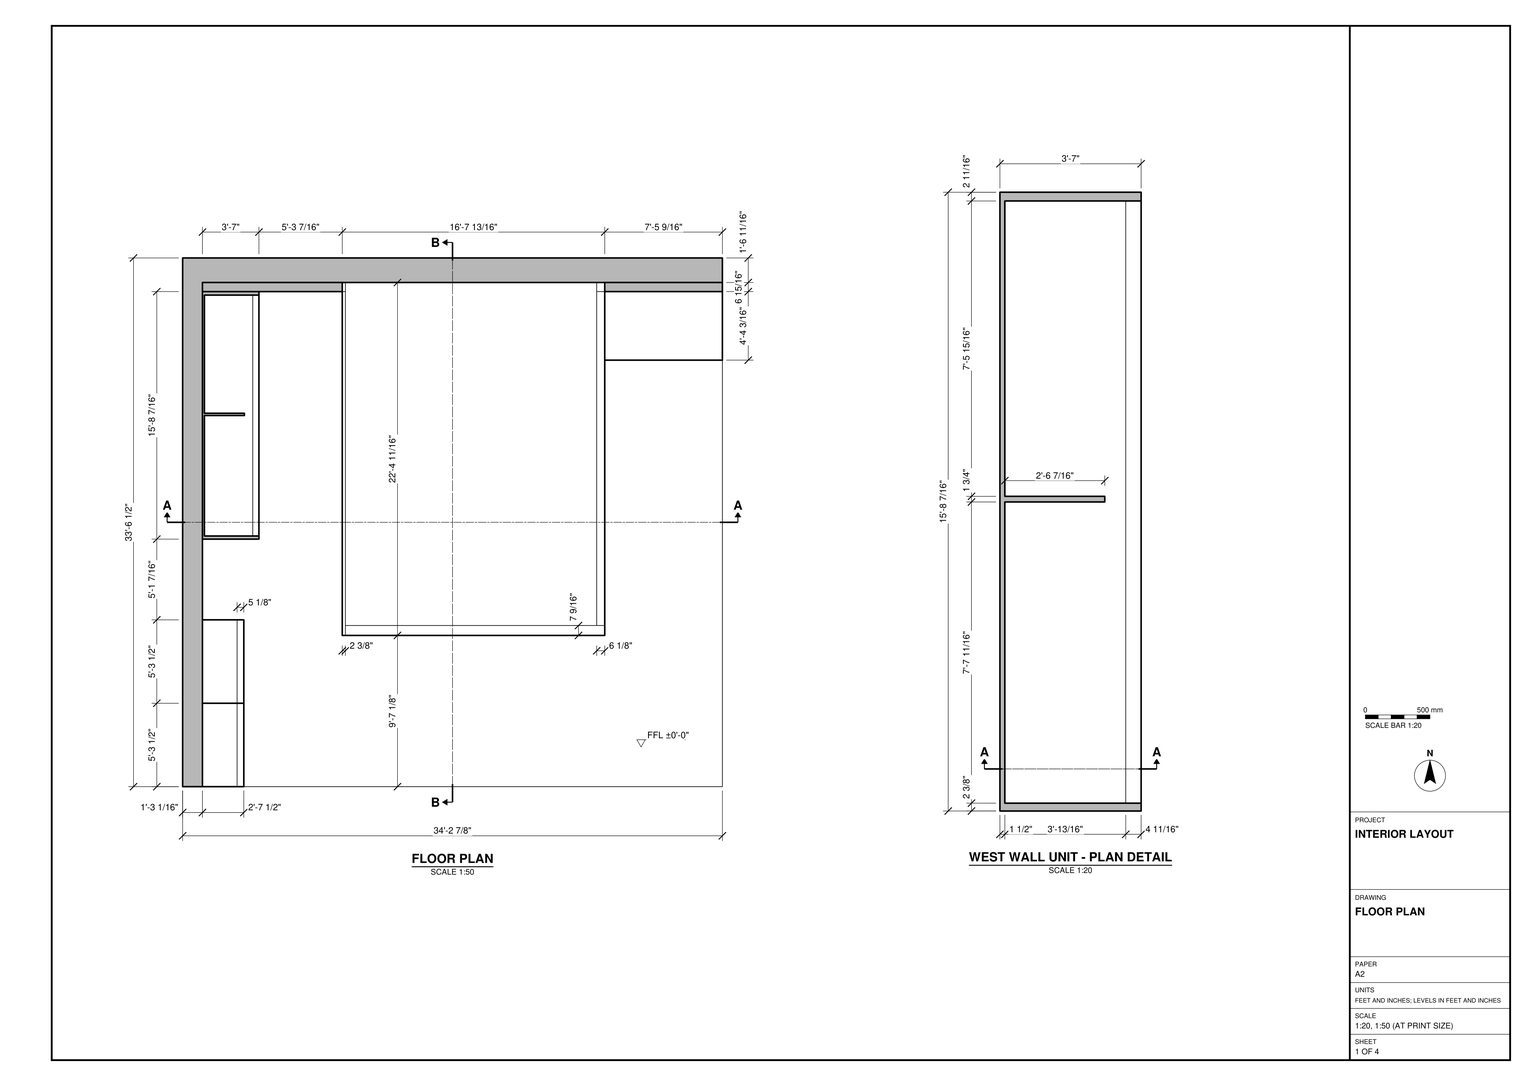
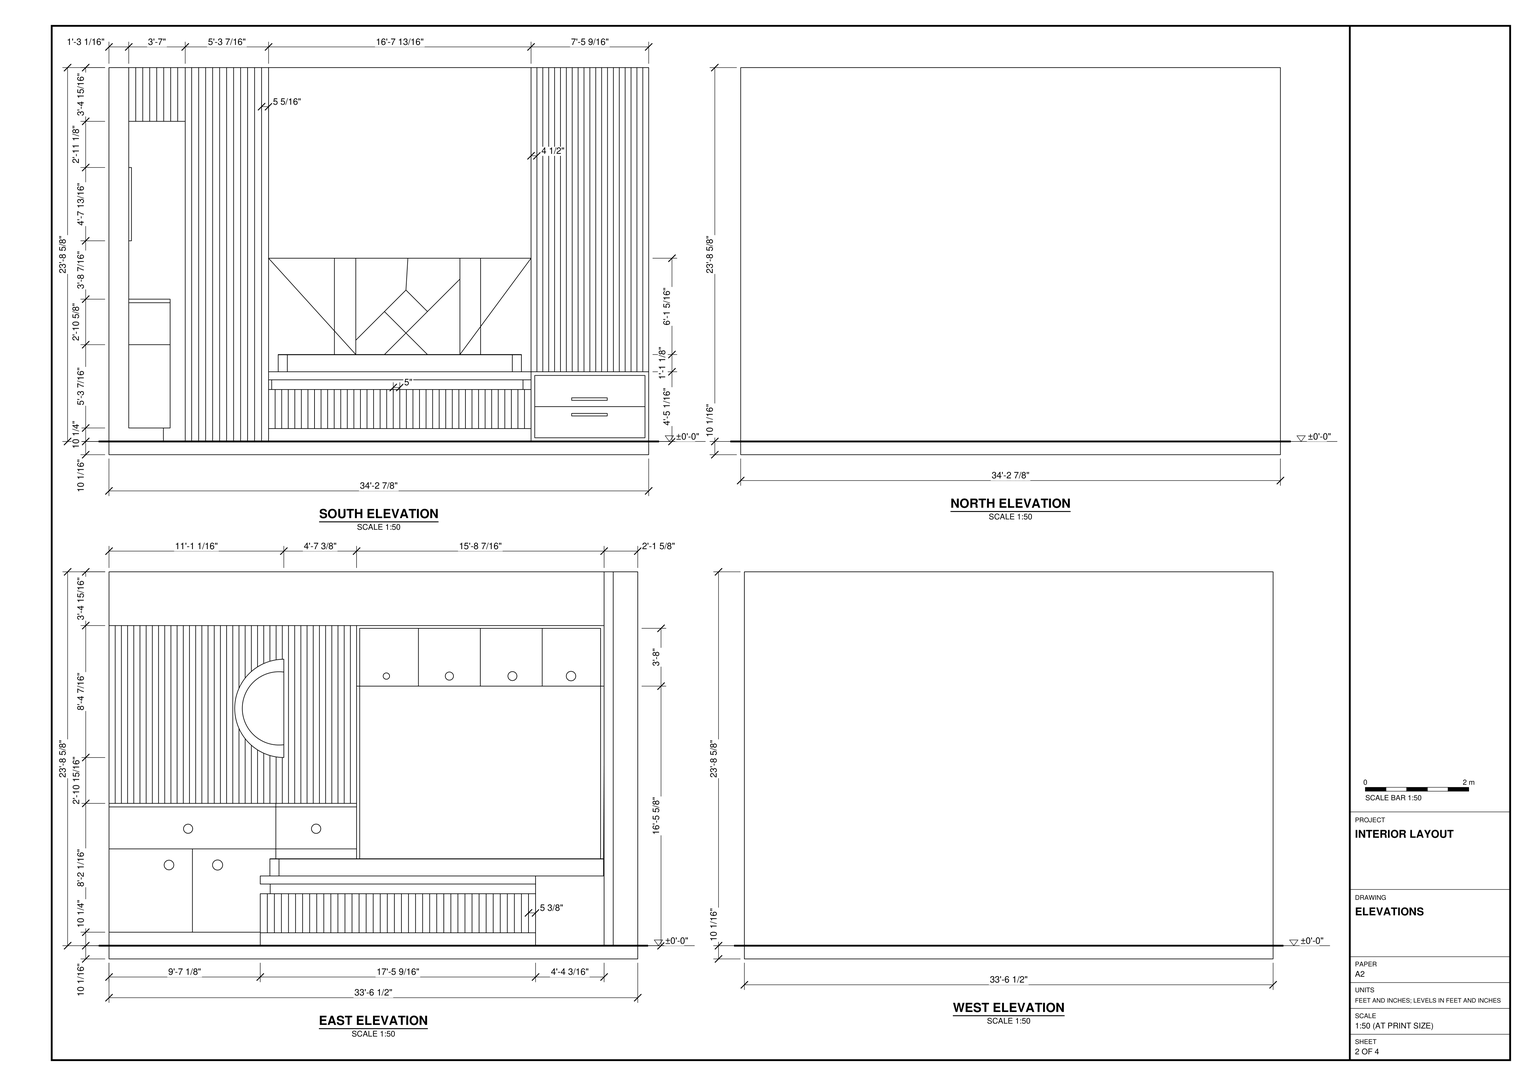
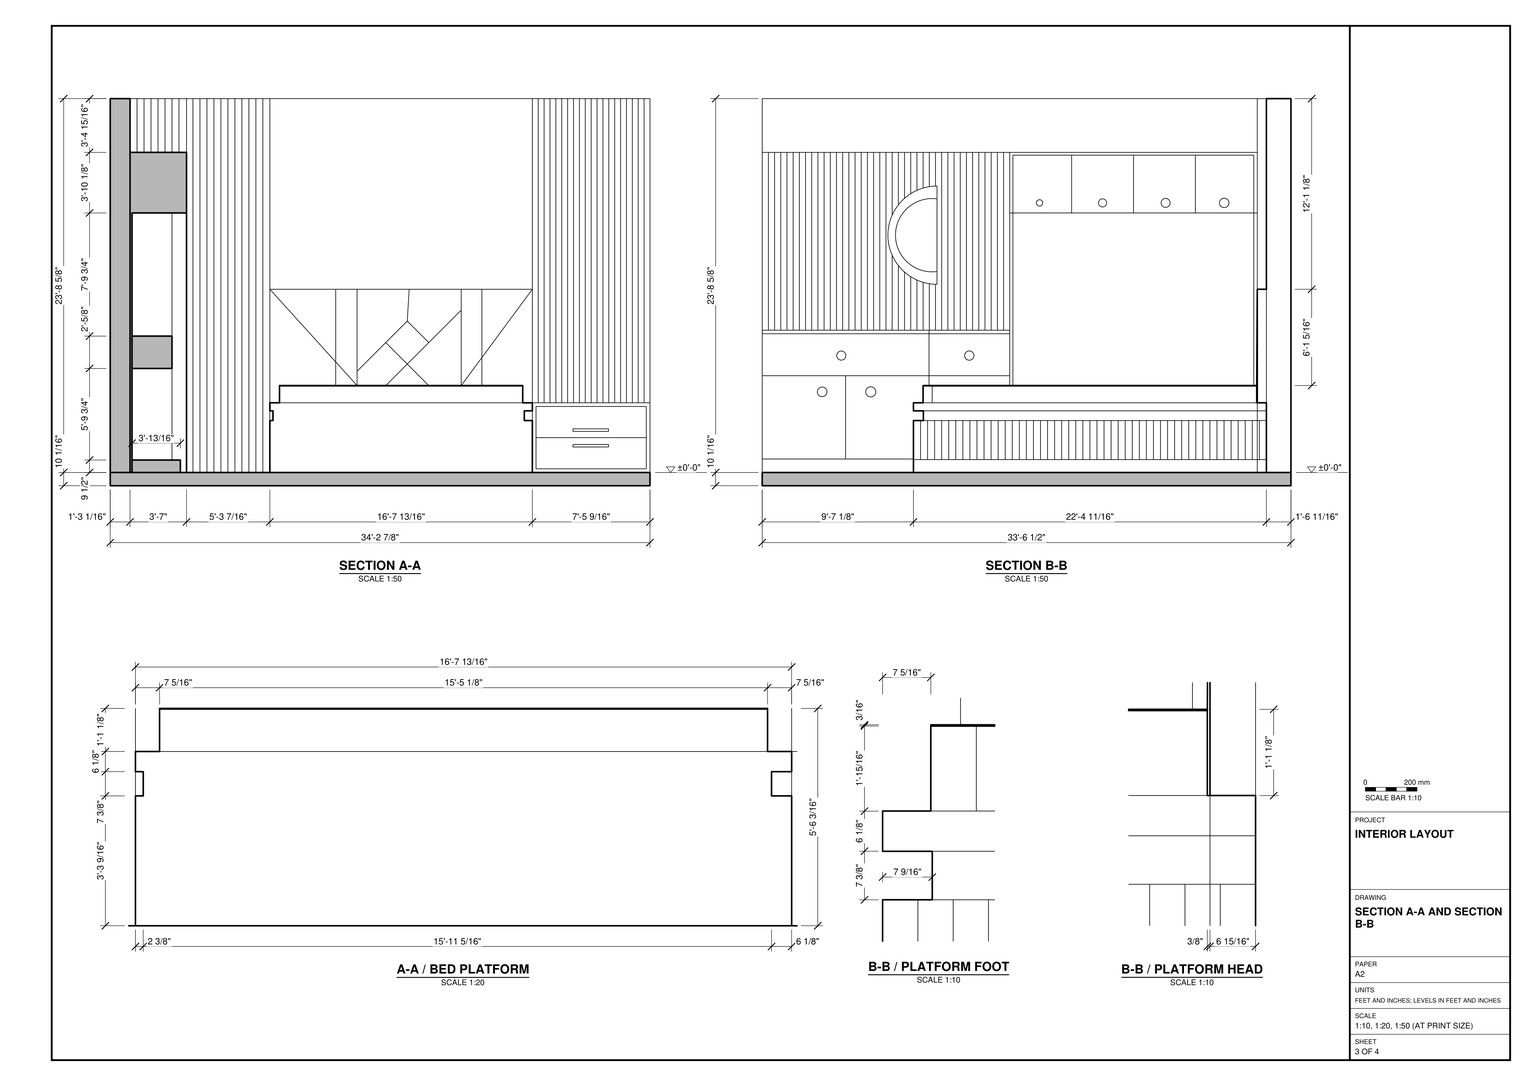
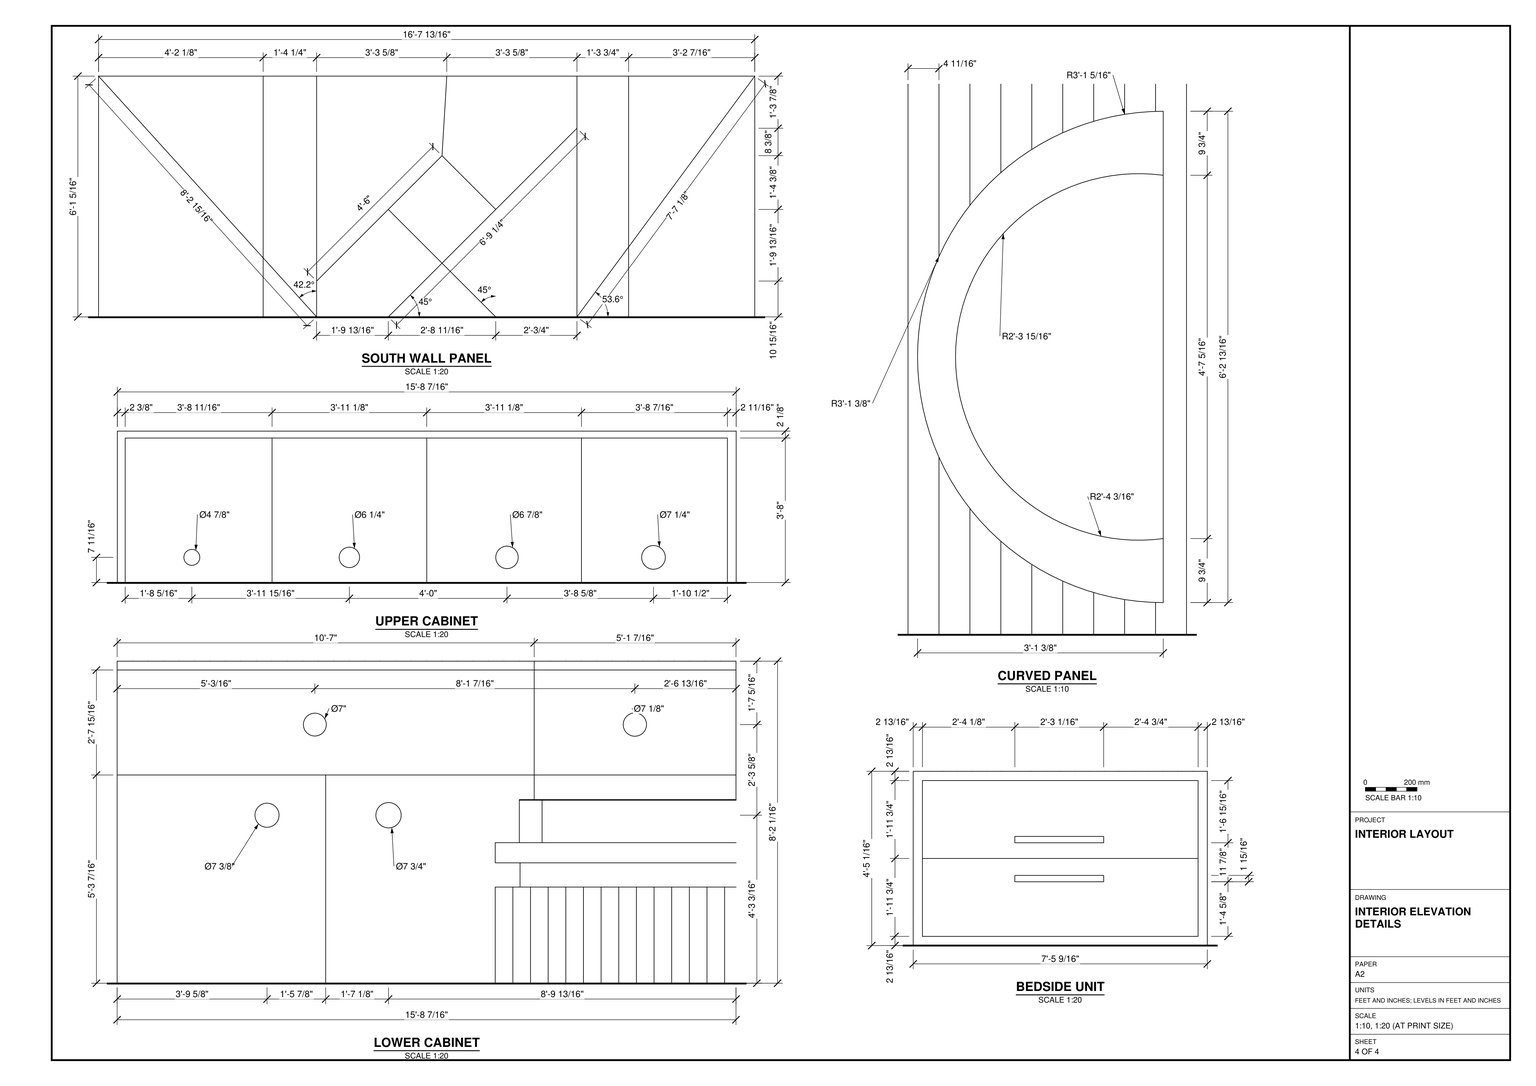
Build the bedroom interior in SketchUp from task_files/diagram_01.pdf. Work in feet and inches. The overall model is 34'-2 7/8" east to west, 33'-6 1/2" north to south and 24'-6 11/16" high. Set the finished floor at ±0'-0". Model the rectangular floor slab and the two walls meeting at the northwest corner. The west wall is 1'-3 1/16" thick and the north wall is 1'-6 11/16" thick. Leave the south and east sides open as drawn.

Place the platform bed with its head against the north wall and its foot facing the open floor to the south. Use the enlarged sections to shape the projecting platform edge, recessed band and inset mattress. Match the vertical divisions on the base, the angular panel pattern above the bed and the narrow vertical panels flanking the headboard. Fit the low drawer cabinet beside the bed. On the west wall, use the plan detail to set out the deep wall unit and its internal division. Use the east elevation to position its upper cupboards and the adjoining storage, vertically divided panel and semicircular feature.

Keep the walls, floor slab and each furniture or joinery piece in separate groups or components, and use components for repeated parts. Decor and loose items may be any suitable library components. Save one SketchUp model as output_files/bedroom_with_a_platform_bed_and_wall_joinery.skp.

# SketchUp Ruby script. Lengths in inches.
U = 1.inch
M = Sketchup.active_model
def pt(a) = Geom::Point3d.new(a.map { |v| v * U })
def face(e, loops, mat)
  f = e.add_face(loops[0].map { |a| pt(a) })
  loops[1..].each { |l| e.add_face(l.map { |a| pt(a) }).erase! }
  f.material = f.back_material = mat if mat
  f
end
# faces: each face lists its corners as indices into pts; further lists are holes
def faces(e, pts, list, mat = nil) = list.each { |f| face(e, (f[0].is_a?(Array) ? f : [f]).map { |l| l.map { |i| pts[i] } }, mat) }
# xy, xz, yz: faces in a plane at the given z, y or x. An outline is a flat list of corners, or four numbers for a rectangle; further outlines are holes
def ring(l) = l.size == 4 ? [[l[0], l[1]], [l[2], l[1]], [l[2], l[3]], [l[0], l[3]]] : l.each_slice(2).to_a
def flat(e, list, mat, &to3) = list.each { |f| face(e, (f[0].is_a?(Array) ? f : [f]).map { |l| ring(l).map { |u, v| to3.(u, v) } }, mat) }
def xy(e, z, list, mat = nil) = flat(e, list, mat) { |x, y| [x, y, z] }
def xz(e, y, list, mat = nil) = flat(e, list, mat) { |x, z| [x, y, z] }
def yz(e, x, list, mat = nil) = flat(e, list, mat) { |y, z| [x, y, z] }
def lines(e, pts, list) = list.each { |a, b| e.add_line(pt(pts[a]), pt(pts[b])) }
# prism: a flat outline (further loops are holes) pulled along v
def prism(e, loops, v, mat = nil)
  f = face(e, loops, mat); d = Geom::Vector3d.new(v.map { |x| x * U })
  f.pushpull(f.normal.samedirection?(d) ? d.length : -d.length)
end
def box(e, o, s, mat = nil) = prism(e, [[o, [o[0] + s[0], o[1], o[2]], [o[0] + s[0], o[1] + s[1], o[2]], [o[0], o[1] + s[1], o[2]]]], [0, 0, s[2]], mat)
def at(x, y, z, deg = 0) = Geom::Transformation.translation(pt([x, y, z])) * Geom::Transformation.rotation(ORIGIN, Z_AXIS, deg.degrees)
def axes(o, x, y, z) = Geom::Transformation.new([*x, 0, *y, 0, *z, 0, *pt(o).to_a, 1])
def part(name) = M.definitions.add(name)
# library, detail: a bought-in or finely detailed component or shape, given as its bounding box
def library(name, o, s) = part(name).tap { |d| box(d.entities, o, s) }
def detail(e, o, s) = box(e.add_group.entities, o, s)
def put(e, d, t, mat = nil) = e.add_instance(d, t).tap { |i| i.material = mat if mat }
def group(e, t, mat = nil) = e.add_group.tap { |g| g.transformation = t; g.material = mat if mat }.entities
root = M.entities
M.materials.add("[0058_Olive]").color = [142, 142, 0]
M.materials.add("[Textile Leaves Green]").color = [226, 227, 196]
M.materials.add("[Translucent Glass Dark Green]").color = [24, 7, 1]
M.materials["[Translucent Glass Dark Green]"].alpha = 0.5
xy(root,0,[[0,0,410.875,402.5]])
xy(root,10.0625,[[0,0,0,402.5,410.875,402.5,410.875,383.8125,15.07,383.8125,15.07,126.99,41.44,126.99,41.44,0],[41.44,0,410.875,0,410.875,324.7,321.32,324.7,321.32,115.125,121.51,115.125,121.51,376.875,58.07,376.875,58.07,188.4375,15.07,188.4375,15.07,126.99,41.44,126.99],[121.51,115.125,321.32,383.8125],[15.07,188.4375,58.07,188.4375,58.07,190.83,16.57,190.83,16.57,374.21,58.07,374.21,58.07,376.875,15.07,376.875],[16.57,190.83,53.38,374.21],
  [53.38,190.83,58.07,374.21],[321.32,324.7,410.875,376.875],[15.07,376.875,121.51,383.8125],[321.32,376.875,410.875,383.8125]])
xy(root,19.54,[[16.57,190.83,53.38,190.83,53.38,374.21,16.57,374.21,16.57,284.27,47,284.27,47,282.52,16.57,282.52],[16.57,282.52,47,284.27]])
xy(root,20.32,[[15.07,0,41.44,63.5],[41.44,0,46.57,63.5],[15.07,63.5,41.44,126.99],[41.44,63.5,46.57,126.99]])
xy(root,49.61,[[121.51,115.125,123.88,376.875],[123.88,115.125,321.32,122.6875],[315.2,122.6875,321.32,376.875],[121.51,376.875,123.88,383.8125],[315.2,376.875,321.32,383.8125]])
xy(root,56.99,[[121.51,115.125,123.88,376.875],[123.88,115.125,321.32,122.6875],[315.2,122.6875,321.32,376.875],[121.51,376.875,123.88,383.8125],[315.2,376.875,321.32,383.8125]])
xy(root,63.125,[[[121.51,115.125,321.32,376.875],[135.78,122.47,134.875,122.53,133.98,122.7,133.125,122.99,132.3125,123.4,131.56,123.9,130.88,124.5,130.28,125.18,129.78,125.93,129.375,126.75,129.08,127.6,128.91,128.49,128.85,129.4,128.85,376.47,313.98,376.47,313.98,129.4,313.92,128.49,313.74,127.6,313.45,126.75,313.05,125.93,312.55,125.18,311.95,124.5,311.27,123.9,310.52,123.4,309.7,122.99,308.84,122.7,307.95,122.53,307.05,122.47]],[321.32,324.7,410.875,376.875],[121.51,376.875,321.32,383.8125]])
xy(root,76.0625,[[135.78,122.47,134.875,122.53,133.98,122.7,133.125,122.99,132.3125,123.4,131.56,123.9,130.88,124.5,130.28,125.18,129.78,125.93,129.375,126.75,129.08,127.6,128.91,128.49,128.85,129.4,128.85,376.47,313.98,376.47,313.98,129.4,313.92,128.49,313.74,127.6,313.45,126.75,313.05,125.93,312.55,125.18,311.95,124.5,311.27,123.9,310.52,123.4,309.7,122.99,308.84,122.7,307.95,122.53,307.05,122.47]])
xy(root,76.25,[[135.78,122.47,307.05,122.47,307.95,122.53,308.84,122.7,309.7,122.99,310.52,123.4,311.27,123.9,311.95,124.5,312.55,125.18,313.05,125.93,313.45,126.75,313.74,127.6,313.92,128.49,313.98,129.4,313.98,376.47,128.85,376.47,128.85,129.4,128.91,128.49,129.08,127.6,129.375,126.75,129.78,125.93,130.28,125.18,130.88,124.5,131.56,123.9,132.3125,123.4,133.125,122.99,133.98,122.7,134.875,122.53]],"[Textile Leaves Green]")
xy(root,83.75,[[15.07,0,46.57,63.5],[15.07,63.5,46.57,126.99],[15.07,126.99,46.57,188.4375]])
xy(root,115.71,[[15.07,0,46.57,188.4375]])
xy(root,118.4,[[15.07,0,46.57,188.4375]])
xy(root,149.57,[[121.51,376.875,321.32,383.8125]])
xy(root,207.66,[[16.57,190.83,58.07,235.55],[16.57,235.55,58.07,282.66],[47,282.66,47,284.28,16.57,284.28,16.57,329.77,58.07,329.77,58.07,282.66],[16.57,329.77,58.07,374.21]])
xy(root,253.77,[[15.07,188.4375,58.07,376.875],[15.07,376.875,20.39,381.1875],[20.39,376.875,25.71,380.6875],[25.71,376.875,31.03,381.0625],[31.03,376.875,36.36,379.625],
  [36.36,376.875,41.68,378.5],[41.68,376.875,47,377.9375],[47,376.875,52.32,377.875],[52.32,376.875,57.64,379.375]])
xy(root,294.6875,[[0,0,15.07,0,15.07,383.8125,410.875,383.8125,410.875,402.5,0,402.5],[15.07,376.875,121.51,383.8125],[321.32,376.875,410.875,383.8125]])
xz(root,0,[[0,0,410.875,10.0625],[0,10.0625,41.44,10.0625,41.44,20.32,15.07,20.32,15.07,294.6875,0,294.6875],[15.07,20.32,46.57,83.75],[15.07,83.75,46.57,115.71],[15.07,115.71,46.57,118.4]])
xz(root,63.5,[[15.07,20.32,46.57,83.75]])
xz(root,115.125,[[121.51,10.0625,321.32,19.88],[121.51,56.99,321.32,63.125]])
xz(root,115.125,[[121.51,19.88,126.5,49.61],[126.5,19.88,131.5,49.61],[131.5,19.88,136.49,49.61],[136.49,19.88,141.49,49.61],[141.49,19.88,146.48,49.61],
  [146.48,19.88,151.48,49.61],[151.48,19.88,156.47,49.61],[156.47,19.88,161.47,49.61],[161.47,19.88,166.46,49.61],[166.46,19.88,171.46,49.61],
  [171.46,19.88,176.46,49.61],[176.46,19.88,181.45,49.61],[181.45,19.88,186.45,49.61],[186.45,19.88,191.44,49.61],[191.44,19.88,196.4375,49.61],
  [196.4375,19.88,201.43,49.61],[201.43,19.88,206.43,49.61],[206.43,19.88,211.42,49.61],[211.42,19.88,216.42,49.61],[216.42,19.88,221.41,49.61],
  [221.41,19.88,226.41,49.61],[226.41,19.88,231.41,49.61],[231.41,19.88,236.4,49.61],[236.4,19.88,241.4,49.61],[241.4,19.88,246.39,49.61],
  [246.39,19.88,251.39,49.61],[251.39,19.88,256.38,49.61],[256.38,19.88,261.38,49.61],[261.38,19.88,266.375,49.61],[266.375,19.88,271.37,49.61],
  [271.37,19.88,276.36,49.61],[276.36,19.88,281.36,49.61],[281.36,19.88,286.35,49.61],[286.35,19.88,291.35,49.61],[291.35,19.88,296.35,49.61],
  [296.35,19.88,301.34,49.61],[301.34,19.88,306.34,49.61],[306.34,19.88,311.33,49.61],[311.33,19.88,316.33,49.61],[316.33,19.88,321.32,49.61]],"[0058_Olive]")
xz(root,122.47,[[135.78,76.0625,307.05,76.25]])
xz(root,122.47,[[135.78,63.125,307.05,76.0625]],"[Textile Leaves Green]")
xz(root,122.6875,[[123.88,49.61,315.2,56.99]])
xz(root,126.99,[[15.07,10.0625,41.44,20.32],[15.07,20.32,46.57,62],[15.07,62,46.57,83.75]])
xz(root,133.07,[[15.07,163.08,17.13,218.39]])
xz(root,188.4375,[[15.07,10.0625,58.07,10.0625,58.07,253.77,15.07,253.77,15.07,118.4,46.57,118.4,46.57,83.75,15.07,83.75],[15.07,83.75,46.57,115.71],[15.07,115.71,46.57,118.4]])
xz(root,190.83,[[16.57,10.0625,53.38,19.54],[53.38,10.0625,53.38,19.54,16.57,19.54,16.57,207.66,58.07,207.66,58.07,10.0625]])
xz(root,284.27,[[16.57,19.54,47,101.27]])
xz(root,284.28,[[16.57,126.41,47,207.66]])
xz(root,324.7,[[[321.32,10.0625,410.875,63.125],[324.13,12.87,408.07,60.32]],[[324.13,12.87,408.07,36.59],[352.26,29.49,379.32,31.43]],[[324.13,36.59,408.07,60.32],[352.26,41.37,379.32,43.31]]])
xz(root,324.7,[[352.26,29.49,379.32,31.43],[352.26,41.37,379.32,43.31]],"[0058_Olive]")
xz(root,374.21,[[16.57,10.0625,53.38,19.54],[53.38,10.0625,58.07,10.0625,58.07,207.66,16.57,207.66,16.57,126.35,47,126.35,47,101.2,16.57,101.2,16.57,19.54,53.38,19.54],[16.57,101.2,47,126.35]])
xz(root,376.47,[[128.85,63.125,313.98,76.0625],[128.85,76.0625,313.98,76.25]])
xz(root,376.875,[[15.07,10.0625,20.39,253.77],[20.39,10.0625,25.71,253.77],[25.71,10.0625,31.03,253.77],[31.03,10.0625,36.36,253.77],[36.36,10.0625,41.68,253.77],
  [41.68,10.0625,47,253.77],[47,10.0625,52.32,253.77],[52.32,10.0625,57.64,253.77],[57.64,10.0625,58.07,253.77],[321.32,10.0625,325.8,63.125],
  [325.8,10.0625,330.28,63.125],[330.28,10.0625,334.76,63.125],[334.76,10.0625,339.23,63.125],[339.23,10.0625,343.71,63.125],[343.71,10.0625,348.1875,63.125],
  [348.1875,10.0625,352.67,63.125],[352.67,10.0625,357.14,63.125],[357.14,10.0625,361.62,63.125],[361.62,10.0625,366.1,63.125],[366.1,10.0625,370.58,63.125],
  [370.58,10.0625,375.05,63.125],[375.05,10.0625,379.53,63.125],[379.53,10.0625,384.01,63.125],[384.01,10.0625,388.49,63.125],[388.49,10.0625,392.96,63.125],
  [392.96,10.0625,397.44,63.125],[397.44,10.0625,401.92,63.125],[401.92,10.0625,406.4,63.125],[406.4,10.0625,410.875,63.125],[121.51,49.61,123.88,56.99],
  [315.2,49.61,321.32,56.99]])
xz(root,376.875,[[58.07,10.0625,62.97,294.6875],[62.97,10.0625,68.29,294.6875],[68.29,10.0625,73.61,294.6875],[73.61,10.0625,78.93,294.6875],[78.93,10.0625,84.25,294.6875],
  [84.25,10.0625,89.57,294.6875],[89.57,10.0625,94.9,294.6875],[94.9,10.0625,100.22,294.6875],[100.22,10.0625,105.54,294.6875],[105.54,10.0625,110.86,294.6875],
  [110.86,10.0625,116.18,294.6875],[116.18,10.0625,121.51,294.6875],[121.51,63.125,321.32,149.57],[321.32,63.125,325.8,294.6875],[325.8,63.125,330.28,294.6875],
  [330.28,63.125,334.76,294.6875],[334.76,63.125,339.23,294.6875],[339.23,63.125,343.71,294.6875],[343.71,63.125,348.1875,294.6875],[348.1875,63.125,352.67,294.6875],
  [352.67,63.125,357.14,294.6875],[357.14,63.125,361.62,294.6875],[361.62,63.125,366.1,294.6875],[366.1,63.125,370.58,294.6875],[370.58,63.125,375.05,294.6875],
  [375.05,63.125,379.53,294.6875],[379.53,63.125,384.01,294.6875],[384.01,63.125,388.49,294.6875],[388.49,63.125,392.96,294.6875],[392.96,63.125,397.44,294.6875],
  [397.44,63.125,401.92,294.6875],[401.92,63.125,406.4,294.6875],[406.4,63.125,410.875,294.6875],[15.07,253.77,20.39,294.6875],[20.39,253.77,25.71,294.6875],
  [25.71,253.77,31.03,294.6875],[31.03,253.77,36.36,294.6875],[36.36,253.77,41.68,294.6875],[41.68,253.77,47,294.6875],[47,253.77,52.32,294.6875],
  [52.32,253.77,58.07,294.6875]],"[0058_Olive]")
xz(root,383.8125,[[15.07,10.0625,15.07,294.6875,121.51,294.6875,121.51,56.99,123.88,56.99,123.88,49.61,121.51,49.61,121.51,10.0625],[121.51,10.0625,321.32,10.0625,321.32,49.61,315.2,49.61,315.2,56.99,321.32,56.99,321.32,63.125,121.51,63.125,121.51,56.99,123.88,56.99,123.88,49.61,121.51,49.61],[321.32,10.0625,321.32,49.61,315.2,49.61,315.2,56.99,321.32,56.99,321.32,294.6875,410.875,294.6875,410.875,10.0625],[121.51,149.57,321.32,294.6875]])
xz(root,402.5,[[0,0,410.875,10.0625],[0,10.0625,410.875,294.6875]])
yz(root,0,[[0,0,402.5,10.0625],[0,10.0625,402.5,294.6875]])
yz(root,15.07,[[126.99,10.0625,188.4375,83.75],[188.4375,10.0625,376.875,253.77],[376.875,10.0625,383.8125,10.0625,383.8125,294.6875,381.1875,294.6875,381.1875,253.77,376.875,253.77],[0,20.32,63.5,83.75],[63.5,20.32,126.99,83.75],
  [0,83.75,126.99,115.71],[126.99,83.75,188.4375,115.71],[0,115.71,126.99,118.4],[126.99,115.71,188.4375,118.4],[133.07,153.33,133.07,163.08,131.91,162.95,131.5,162.91,129.91,162.83,128.33,162.85,127.2,162.92,126.75,162.95,125.17,163.14,123.61,163.42,122.48,163.69,122.07,163.79,120.55,164.25,119.0625,164.79,117.77,165.35,117.61,165.42,116.1875,166.13,114.8125,166.91,113.48,167.78,113.0625,168.09,112.21,168.72,110.98,169.73,109.82,170.8,108.72,171.94,108.35,172.37,107.6875,173.15,106.72,174.41,105.83,175.72,105.02,177.08,104.28,178.48,103.64,179.89,103.625,179.92,103.05,181.4,102.57,182.91,102.17,184.44,101.85,186,101.63,187.57,101.49,189.15,101.45,190.73,101.49,192.32,101.63,193.9,101.85,195.47,102.17,197.02,102.57,198.55,103.05,200.0625,103.625,201.54,103.64,201.57,104.28,202.98,105.02,204.39,105.83,205.75,106.72,207.06,107.6875,208.32,108.35,209.09,108.72,209.52,109.82,210.66,110.98,211.74,112.21,212.75,113.0625,213.375,113.48,213.6875,114.8125,214.55,116.1875,215.34,117.61,216.04,117.77,216.12,119.0625,216.67,120.55,217.21,122.07,217.67,122.48,217.77,123.61,218.04,125.17,218.32,126.75,218.52,127.2,218.54,128.33,218.62,129.91,218.63,131.5,218.55,131.91,218.51,133.07,218.39,133.07,228.14,131.91,228.11,131.11,228.09,129.16,227.93,127.22,227.68,127.2,227.67,125.3,227.32,123.39,226.86,122.48,226.6,121.51,226.31,119.67,225.65,117.86,224.9,117.77,224.86,116.09,224.0625,114.37,223.125,113.0625,222.33,112.7,222.1,111.09,220.99,109.53,219.8,108.35,218.79,108.04,218.53,106.62,217.18,105.27,215.76,104,214.27,103.64,213.8,102.81,212.72,101.7,211.1,100.68,209.44,99.74,207.71,98.93,206.01,98.9,205.95,98.15,204.14,97.5,202.29,96.94,200.41,96.48,198.51,96.125,196.58,95.87,194.64,95.72,192.69,95.67,190.73,95.72,188.77,95.87,186.82,96.125,184.88,96.48,182.95,96.94,181.05,97.5,179.17,98.15,177.33,98.9,175.52,98.93,175.46,99.74,173.75,100.68,172.03,101.7,170.36,102.81,168.75,103.64,167.66,104,167.19,105.27,165.7,106.62,164.28,108.04,162.93,108.35,162.67,109.53,161.66,111.09,160.47,112.7,159.36,113.0625,159.14,114.37,158.34,116.09,157.4,117.77,156.6,117.86,156.56,119.67,155.81,121.51,155.16,122.48,154.87,123.39,154.6,125.3,154.14,127.2,153.79,127.22,153.79,129.16,153.53,131.11,153.38,131.91,153.36],
  [129.91,162.83,128.33,162.85,127.2,162.92,127.2,218.54,128.33,218.62,129.91,218.63,131.5,218.55,131.91,218.51,131.91,162.95,131.5,162.91],[127.2,162.92,126.75,162.95,125.17,163.14,123.61,163.42,122.48,163.69,122.48,217.77,123.61,218.04,125.17,218.32,126.75,218.52,127.2,218.54],[131.91,162.95,131.91,218.51,133.07,218.39,133.07,163.08],[122.48,163.69,122.07,163.79,120.55,164.25,119.0625,164.79,117.77,165.35,117.77,216.12,119.0625,216.67,120.55,217.21,122.07,217.67,122.48,217.77],[117.77,165.35,117.61,165.42,116.1875,166.13,114.8125,166.91,113.48,167.78,113.0625,168.09,113.0625,213.375,113.48,213.6875,114.8125,214.55,116.1875,215.34,117.61,216.04,117.77,216.12],
  [113.0625,168.09,112.21,168.72,110.98,169.73,109.82,170.8,108.72,171.94,108.35,172.37,108.35,209.09,108.72,209.52,109.82,210.66,110.98,211.74,112.21,212.75,113.0625,213.375],[108.35,172.37,107.6875,173.15,106.72,174.41,105.83,175.72,105.02,177.08,104.28,178.48,103.64,179.89,103.64,201.57,104.28,202.98,105.02,204.39,105.83,205.75,106.72,207.06,107.6875,208.32,108.35,209.09],[103.64,179.89,103.625,179.92,103.05,181.4,102.57,182.91,102.17,184.44,101.85,186,101.63,187.57,101.49,189.15,101.45,190.73,101.49,192.32,101.63,193.9,101.85,195.47,102.17,197.02,102.57,198.55,103.05,200.0625,103.625,201.54,103.64,201.57],[0,253.77,376.875,294.6875],[376.875,253.77,381.1875,294.6875]])
yz(root,15.07,[[0,118.4,4.71,253.77],[4.71,118.4,9.42,253.77],[9.42,118.4,14.13,253.77],[14.13,118.4,18.84,253.77],[18.84,118.4,23.55,253.77],
  [23.55,118.4,28.27,253.77],[28.27,118.4,32.98,253.77],[32.98,118.4,37.6875,253.77],[37.6875,118.4,42.4,253.77],[42.4,118.4,47.11,253.77],
  [47.11,118.4,51.82,253.77],[51.82,118.4,56.53,253.77],[56.53,118.4,61.24,253.77],[61.24,118.4,65.95,253.77],[65.95,118.4,70.66,253.77],
  [70.66,118.4,75.375,253.77],[75.375,118.4,80.09,253.77],[80.09,118.4,84.8,253.77],[84.8,118.4,89.51,253.77],[89.51,118.4,94.22,253.77],
  [94.22,118.4,98.93,118.4,98.93,175.46,98.9,175.52,98.15,177.33,97.5,179.17,96.94,181.05,96.48,182.95,96.125,184.88,95.87,186.82,95.72,188.77,95.67,190.73,95.72,192.69,95.87,194.64,96.125,196.58,96.48,198.51,96.94,200.41,97.5,202.29,98.15,204.14,98.9,205.95,98.93,206.01,98.93,253.77,94.22,253.77],[98.93,118.4,103.64,118.4,103.64,167.66,102.81,168.75,101.7,170.36,100.68,172.03,99.74,173.75,98.93,175.46],[103.64,118.4,108.35,118.4,108.35,162.67,108.04,162.93,106.62,164.28,105.27,165.7,104,167.19,103.64,167.66],[108.35,118.4,113.0625,118.4,113.0625,159.14,112.7,159.36,111.09,160.47,109.53,161.66,108.35,162.67],[113.0625,118.4,117.77,118.4,117.77,156.6,116.09,157.4,114.37,158.34,113.0625,159.14],
  [117.77,118.4,122.48,118.4,122.48,154.87,121.51,155.16,119.67,155.81,117.86,156.56,117.77,156.6],[122.48,118.4,127.2,118.4,127.2,153.79,125.3,154.14,123.39,154.6,122.48,154.87],[127.2,118.4,131.91,118.4,131.91,153.36,131.11,153.38,129.16,153.53,127.22,153.79,127.2,153.79],[131.91,118.4,136.62,118.4,136.62,253.77,131.91,253.77,131.91,228.11,133.07,228.14,133.07,153.33,131.91,153.36],[136.62,118.4,141.33,253.77],
  [141.33,118.4,146.04,253.77],[146.04,118.4,150.75,253.77],[150.75,118.4,155.46,253.77],[155.46,118.4,160.17,253.77],[160.17,118.4,164.88,253.77],
  [164.88,118.4,169.59,253.77],[169.59,118.4,174.3,253.77],[174.3,118.4,179.02,253.77],[179.02,118.4,183.73,253.77],[183.73,118.4,188.4375,253.77],
  [98.93,206.01,99.74,207.71,100.68,209.44,101.7,211.1,102.81,212.72,103.64,213.8,103.64,253.77,98.93,253.77],[103.64,213.8,104,214.27,105.27,215.76,106.62,217.18,108.04,218.53,108.35,218.79,108.35,253.77,103.64,253.77],[108.35,218.79,109.53,219.8,111.09,220.99,112.7,222.1,113.0625,222.33,113.0625,253.77,108.35,253.77],[113.0625,222.33,114.37,223.125,116.09,224.0625,117.77,224.86,117.77,253.77,113.0625,253.77],[117.77,224.86,117.86,224.9,119.67,225.65,121.51,226.31,122.48,226.6,122.48,253.77,117.77,253.77],
  [122.48,226.6,123.39,226.86,125.3,227.32,127.2,227.67,127.2,253.77,122.48,253.77],[127.2,227.67,127.22,227.68,129.16,227.93,131.11,228.09,131.91,228.11,131.91,253.77,127.2,253.77]],"[0058_Olive]")
yz(root,16.57,[[190.83,10.0625,374.21,19.54],[190.83,19.54,282.52,19.54,282.57,89.21,190.83,89.27],[284.27,19.54,374.21,19.54,374.21,101.2,284.27,101.27],[282.57,89.21,190.83,89.27,190.85,113.91,282.59,113.84],[190.83,89.27,190.85,113.91,190.83,113.91],
  [374.21,101.2,284.27,101.27,284.28,126.41,374.21,126.35],[374.21,101.2,374.23,126.35,374.21,126.35],[282.59,113.84,282.66,207.66,190.83,207.66,190.83,113.91,190.85,113.91],[374.21,126.35,374.21,207.66,284.28,207.66,284.28,126.41]])
yz(root,17.13,[[129.91,162.83,131.5,162.91,133.07,163.08,133.07,218.39,131.5,218.55,129.91,218.63,128.33,218.62,126.75,218.52,125.17,218.32,123.61,218.04,122.07,217.67,120.55,217.21,119.0625,216.67,117.61,216.04,116.1875,215.34,114.8125,214.55,113.48,213.6875,112.21,212.75,110.98,211.74,109.82,210.66,108.72,209.52,107.6875,208.32,106.72,207.06,105.83,205.75,105.02,204.39,104.28,202.98,103.625,201.54,103.05,200.0625,102.57,198.55,102.17,197.02,101.85,195.47,101.63,193.9,101.49,192.32,101.45,190.73,101.49,189.15,101.63,187.57,101.85,186,102.17,184.44,102.57,182.91,103.05,181.4,103.625,179.92,104.28,178.48,105.02,177.08,105.83,175.72,106.72,174.41,107.6875,173.15,108.72,171.94,109.82,170.8,110.98,169.73,112.21,168.72,113.48,167.78,114.8125,166.91,116.1875,166.13,117.61,165.42,119.0625,164.79,120.55,164.25,122.07,163.79,123.61,163.42,125.17,163.14,126.75,162.95,128.33,162.85]])
yz(root,41.44,[[0,10.0625,126.99,20.32]])
yz(root,46.57,[[[0,20.32,63.5,83.75],[45.63,67.8,44.68,67.93,43.79,68.3,43.03,68.88,42.44,69.65,42.07,70.54,41.95,71.49,42.07,72.44,42.44,73.33,43.03,74.1,43.79,74.68,44.68,75.05,45.63,75.18,46.59,75.05,47.48,74.68,48.24,74.1,48.83,73.33,49.2,72.44,49.32,71.49,49.2,70.54,48.83,69.65,48.24,68.88,47.48,68.3,46.59,67.93]],[[63.5,20.32,126.99,83.75],[82.64,67.61,81.63,67.75,80.7,68.13,79.9,68.75,79.28,69.55,78.89,70.49,78.76,71.49,78.89,72.49,79.28,73.43,79.9,74.23,80.7,74.85,81.63,75.23,82.64,75.36,83.64,75.23,84.57,74.85,85.375,74.23,85.99,73.43,86.38,72.49,86.51,71.49,86.38,70.49,85.99,69.55,85.375,68.75,84.57,68.13,83.64,67.75]],[[0,83.75,126.99,115.71],[60.2,95.59,59.29,95.71,58.45,96.0625,57.72,96.62,57.17,97.34,56.82,98.1875,56.7,99.09,56.82,100,57.17,100.84,57.72,101.57,58.45,102.125,59.29,102.47,60.2,102.59,61.11,102.47,61.95,102.125,62.67,101.57,63.23,100.84,63.58,100,63.7,99.09,63.58,98.1875,63.23,97.34,62.67,96.62,61.95,96.0625,61.11,95.71]],[[126.99,83.75,188.4375,115.71],[157.65,95.53,156.72,95.65,155.86,96.01,155.125,96.57,154.56,97.3125,154.2,98.17,154.08,99.09,154.2,100.01,154.56,100.875,155.125,101.61,155.86,102.18,156.72,102.53,157.65,102.66,158.57,102.53,159.43,102.18,160.16,101.61,160.73,100.875,161.09,100.01,161.21,99.09,161.09,98.17,160.73,97.3125,160.16,96.57,159.43,96.01,158.57,95.65]],[0,115.71,126.99,118.4],
  [126.99,115.71,188.4375,118.4]])
yz(root,46.57,[[82.64,67.61,83.64,67.75,84.57,68.13,85.375,68.75,85.99,69.55,86.38,70.49,86.51,71.49,86.38,72.49,85.99,73.43,85.375,74.23,84.57,74.85,83.64,75.23,82.64,75.36,81.63,75.23,80.7,74.85,79.9,74.23,79.28,73.43,78.89,72.49,78.76,71.49,78.89,70.49,79.28,69.55,79.9,68.75,80.7,68.13,81.63,67.75],[45.63,67.8,46.59,67.93,47.48,68.3,48.24,68.88,48.83,69.65,49.2,70.54,49.32,71.49,49.2,72.44,48.83,73.33,48.24,74.1,47.48,74.68,46.59,75.05,45.63,75.18,44.68,75.05,43.79,74.68,43.03,74.1,42.44,73.33,42.07,72.44,41.95,71.49,42.07,70.54,42.44,69.65,43.03,68.88,43.79,68.3,44.68,67.93],[157.65,95.53,158.57,95.65,159.43,96.01,160.16,96.57,160.73,97.3125,161.09,98.17,161.21,99.09,161.09,100.01,160.73,100.875,160.16,101.61,159.43,102.18,158.57,102.53,157.65,102.66,156.72,102.53,155.86,102.18,155.125,101.61,154.56,100.875,154.2,100.01,154.08,99.09,154.2,98.17,154.56,97.3125,155.125,96.57,155.86,96.01,156.72,95.65],[60.2,95.59,61.11,95.71,61.95,96.0625,62.67,96.62,63.23,97.34,63.58,98.1875,63.7,99.09,63.58,100,63.23,100.84,62.67,101.57,61.95,102.125,61.11,102.47,60.2,102.59,59.29,102.47,58.45,102.125,57.72,101.57,57.17,100.84,56.82,100,56.7,99.09,56.82,98.1875,57.17,97.34,57.72,96.62,58.45,96.0625,59.29,95.71]],"[0058_Olive]")
yz(root,47,[[282.57,89.21,282.59,113.84,190.85,113.91,190.83,89.27],[374.21,101.2,374.21,126.35,284.28,126.41,284.27,101.27],[377.875,253.77,377.9375,294.6875]])
yz(root,47,[[282.52,19.54,284.27,19.54,284.27,101.27,284.28,126.41,284.28,207.66,282.66,207.66,282.59,113.84,282.57,89.21]],"[0058_Olive]")
yz(root,53.38,[[190.83,10.0625,374.21,19.54]])
yz(root,58.07,[[188.4375,207.66,190.83,207.66,190.83,251.66,374.21,251.66,374.21,207.66,376.875,207.66,376.875,253.77,188.4375,253.77],[[190.83,207.66,235.55,251.66],[211.125,212.89,210.49,212.97,209.9,213.21,209.4,213.6,209.01,214.1,208.77,214.69,208.6875,215.32,208.77,215.95,209.01,216.54,209.4,217.05,209.9,217.43,210.49,217.68,211.125,217.76,211.75,217.68,212.34,217.43,212.85,217.05,213.23,216.54,213.48,215.95,213.5625,215.32,213.48,214.69,213.23,214.1,212.85,213.6,212.34,213.21,211.75,212.97]],[[235.55,207.66,282.66,251.66],[259.09,212.2,258.28,212.3,257.52,212.62,256.88,213.11,256.38,213.76,256.07,214.51,255.96,215.32,256.07,216.13,256.38,216.89,256.88,217.53,257.52,218.03,258.28,218.34,259.09,218.45,259.9,218.34,260.65,218.03,261.3,217.53,261.79,216.89,262.11,216.13,262.21,215.32,262.11,214.51,261.79,213.76,261.3,213.11,260.65,212.62,259.9,212.3]],[[282.66,207.66,329.77,251.66],[307.09,211.89,306.2,212,305.37,212.35,304.65,212.89,304.11,213.6,303.76,214.43,303.65,215.32,303.76,216.21,304.11,217.04,304.65,217.75,305.37,218.3,306.2,218.64,307.09,218.76,307.97,218.64,308.8,218.3,309.52,217.75,310.0625,217.04,310.41,216.21,310.52,215.32,310.41,214.43,310.0625,213.6,309.52,212.89,308.8,212.35,307.97,212]],[[329.77,207.66,374.21,251.66],[351.7,211.7,350.76,211.82,349.88,212.18,349.13,212.76,348.56,213.51,348.19,214.39,348.07,215.32,348.19,216.26,348.56,217.14,349.13,217.89,349.88,218.46,350.76,218.82,351.7,218.95,352.63,218.82,353.51,218.46,354.26,217.89,354.83,217.14,355.2,216.26,355.32,215.32,355.2,214.39,354.83,213.51,354.26,212.76,353.51,212.18,352.63,211.82]]])
yz(root,58.07,[[188.4375,10.0625,190.83,207.66],[374.21,10.0625,376.875,207.66],[351.7,211.7,352.63,211.82,353.51,212.18,354.26,212.76,354.83,213.51,355.2,214.39,355.32,215.32,355.2,216.26,354.83,217.14,354.26,217.89,353.51,218.46,352.63,218.82,351.7,218.95,350.76,218.82,349.88,218.46,349.13,217.89,348.56,217.14,348.19,216.26,348.07,215.32,348.19,214.39,348.56,213.51,349.13,212.76,349.88,212.18,350.76,211.82],[307.09,211.89,307.97,212,308.8,212.35,309.52,212.89,310.0625,213.6,310.41,214.43,310.52,215.32,310.41,216.21,310.0625,217.04,309.52,217.75,308.8,218.3,307.97,218.64,307.09,218.76,306.2,218.64,305.37,218.3,304.65,217.75,304.11,217.04,303.76,216.21,303.65,215.32,303.76,214.43,304.11,213.6,304.65,212.89,305.37,212.35,306.2,212],[259.09,212.2,259.9,212.3,260.65,212.62,261.3,213.11,261.79,213.76,262.11,214.51,262.21,215.32,262.11,216.13,261.79,216.89,261.3,217.53,260.65,218.03,259.9,218.34,259.09,218.45,258.28,218.34,257.52,218.03,256.88,217.53,256.38,216.89,256.07,216.13,255.96,215.32,256.07,214.51,256.38,213.76,256.88,213.11,257.52,212.62,258.28,212.3],
  [211.125,212.89,211.75,212.97,212.34,213.21,212.85,213.6,213.23,214.1,213.48,214.69,213.5625,215.32,213.48,215.95,213.23,216.54,212.85,217.05,212.34,217.43,211.75,217.68,211.125,217.76,210.49,217.68,209.9,217.43,209.4,217.05,209.01,216.54,208.77,215.95,208.6875,215.32,208.77,214.69,209.01,214.1,209.4,213.6,209.9,213.21,210.49,212.97]],"[0058_Olive]")
yz(root,58.07,[[190.83,10.0625,374.21,207.66]],"[Translucent Glass Dark Green]")
yz(root,121.51,[[115.125,10.0625,376.875,19.88],[376.875,10.0625,383.8125,19.88],[115.125,19.88,120.5,49.61],[120.5,19.88,125.87,49.61],[125.87,19.88,131.25,49.61],
  [131.25,19.88,136.62,49.61],[136.62,19.88,141.99,49.61],[141.99,19.88,147.37,49.61],[147.37,19.88,152.74,49.61],[152.74,19.88,158.12,49.61],
  [158.12,19.88,163.49,49.61],[163.49,19.88,168.86,49.61],[168.86,19.88,174.24,49.61],[174.24,19.88,179.61,49.61],[179.61,19.88,184.98,49.61],
  [184.98,19.88,190.36,49.61],[190.36,19.88,195.73,49.61],[195.73,19.88,201.1,49.61],[201.1,19.88,206.48,49.61],[206.48,19.88,211.85,49.61],
  [211.85,19.88,217.23,49.61],[217.23,19.88,222.6,49.61],[222.6,19.88,227.97,49.61],[227.97,19.88,233.35,49.61],[233.35,19.88,238.72,49.61],
  [238.72,19.88,244.1,49.61],[244.1,19.88,249.47,49.61],[249.47,19.88,254.84,49.61],[254.84,19.88,260.22,49.61],[260.22,19.88,265.59,49.61],
  [265.59,19.88,270.96,49.61],[270.96,19.88,276.34,49.61],[276.34,19.88,281.71,49.61],[281.71,19.88,287.08,49.61],[287.08,19.88,292.46,49.61],
  [292.46,19.88,297.83,49.61],[297.83,19.88,303.21,49.61],[303.21,19.88,308.58,49.61],[308.58,19.88,313.95,49.61],[313.95,19.88,319.33,49.61],
  [319.33,19.88,324.7,49.61],[324.7,19.88,330.08,49.61],[330.08,19.88,335.45,49.61],[335.45,19.88,340.82,49.61],[340.82,19.88,346.2,49.61],
  [346.2,19.88,351.57,49.61],[351.57,19.88,356.94,49.61],[356.94,19.88,362.32,49.61],[362.32,19.88,367.69,49.61],[367.69,19.88,373.07,49.61],
  [373.07,19.88,376.875,49.61],[376.875,19.88,378.4375,49.61],[378.4375,19.88,383.8125,49.61],[115.125,56.99,376.875,63.125],[376.875,56.99,383.8125,63.125],
  [376.875,63.125,383.8125,149.57],[376.875,149.57,383.8125,294.6875]])
yz(root,123.88,[[122.6875,49.61,376.875,56.99],[376.875,49.61,383.8125,56.99]])
yz(root,128.85,[[129.4,76.0625,376.47,76.25]])
yz(root,128.85,[[129.4,63.125,376.47,76.0625]],"[Textile Leaves Green]")
yz(root,313.98,[[129.4,76.0625,376.47,76.25]])
yz(root,313.98,[[129.4,63.125,376.47,76.0625]],"[Textile Leaves Green]")
yz(root,315.2,[[122.6875,49.61,376.875,56.99],[376.875,49.61,383.8125,56.99]])
yz(root,321.32,[[115.125,10.0625,324.7,19.88],[324.7,10.0625,376.875,19.88],[376.875,10.0625,383.8125,19.88],[324.7,19.88,330.08,49.61],[330.08,19.88,335.45,49.61],
  [330.08,19.88,373.07,49.61],[335.45,19.88,340.82,49.61],[340.82,19.88,346.2,49.61],[346.2,19.88,351.57,49.61],[351.57,19.88,356.94,49.61],
  [356.94,19.88,362.32,49.61],[362.32,19.88,367.69,49.61],[367.69,19.88,373.07,49.61],[373.07,19.88,376.875,49.61],[376.875,19.88,378.4375,49.61],
  [378.4375,19.88,383.8125,49.61],[324.7,49.61,376.875,56.99],[115.125,56.99,324.7,63.125],[324.7,56.99,376.875,63.125],[376.875,56.99,383.8125,63.125],
  [376.875,63.125,383.8125,149.57],[376.875,149.57,383.8125,294.6875]])
yz(root,321.32,[[115.125,19.88,120.5,49.61],[120.5,19.88,125.87,49.61],[125.87,19.88,131.25,49.61],[131.25,19.88,136.62,49.61],[136.62,19.88,141.99,49.61],
  [141.99,19.88,147.37,49.61],[147.37,19.88,152.74,49.61],[152.74,19.88,158.12,49.61],[158.12,19.88,163.49,49.61],[163.49,19.88,168.86,49.61],
  [168.86,19.88,174.24,49.61],[174.24,19.88,179.61,49.61],[179.61,19.88,184.98,49.61],[184.98,19.88,190.36,49.61],[190.36,19.88,195.73,49.61],
  [195.73,19.88,201.1,49.61],[201.1,19.88,206.48,49.61],[206.48,19.88,211.85,49.61],[211.85,19.88,217.23,49.61],[217.23,19.88,222.6,49.61],
  [222.6,19.88,227.97,49.61],[227.97,19.88,233.35,49.61],[233.35,19.88,238.72,49.61],[238.72,19.88,244.1,49.61],[244.1,19.88,249.47,49.61],
  [249.47,19.88,254.84,49.61],[254.84,19.88,260.22,49.61],[260.22,19.88,265.59,49.61],[265.59,19.88,270.96,49.61],[270.96,19.88,276.34,49.61],
  [276.34,19.88,281.71,49.61],[281.71,19.88,287.09,49.61],[287.09,19.88,292.46,49.61],[292.46,19.88,297.83,49.61],[297.83,19.88,303.21,49.61],
  [303.21,19.88,308.58,49.61],[308.58,19.88,313.95,49.61],[313.95,19.88,319.33,49.61],[319.33,19.88,324.7,49.61]],"[0058_Olive]")
yz(root,410.875,[[0,0,402.5,10.0625],[324.7,10.0625,376.875,63.125],[376.875,10.0625,383.8125,294.6875],[383.8125,10.0625,402.5,294.6875]])
p = [[16.57,282.57,89.21],[16.57,282.52,19.54],[47,282.52,19.54],[47,282.57,89.21],[134.875,122.53,76.0625],[133.98,122.7,76.0625],
  [133.98,122.7,63.125],[134.875,122.53,63.125],[135.78,122.47,76.0625],[135.78,122.47,63.125],[307.95,122.53,76.0625],[307.05,122.47,76.0625],
  [307.05,122.47,63.125],[307.95,122.53,63.125],[308.84,122.7,76.0625],[308.84,122.7,63.125],[133.125,122.99,76.0625],[133.125,122.99,63.125],
  [309.7,122.99,76.0625],[309.7,122.99,63.125],[132.3125,123.4,76.0625],[132.3125,123.4,63.125],[310.52,123.4,76.0625],[310.52,123.4,63.125],
  [131.56,123.9,76.0625],[131.56,123.9,63.125],[311.27,123.9,76.0625],[311.27,123.9,63.125],[130.88,124.5,76.0625],[130.88,124.5,63.125],
  [311.95,124.5,76.0625],[311.95,124.5,63.125],[130.28,125.18,76.0625],[130.28,125.18,63.125],[312.55,125.18,76.0625],[312.55,125.18,63.125],
  [129.78,125.93,76.0625],[129.78,125.93,63.125],[313.05,125.93,76.0625],[313.05,125.93,63.125],[129.375,126.75,76.0625],[129.375,126.75,63.125],
  [313.45,126.75,76.0625],[313.45,126.75,63.125],[129.08,127.6,76.0625],[129.08,127.6,63.125],[313.74,127.6,76.0625],[313.74,127.6,63.125],
  [128.91,128.49,76.0625],[128.91,128.49,63.125],[313.92,128.49,76.0625],[313.92,128.49,63.125],[128.85,129.4,76.0625],[128.85,129.4,63.125],
  [313.98,129.4,76.0625],[313.98,129.4,63.125],[134.875,122.53,76.25],[133.98,122.7,76.25],[135.78,122.47,76.25],[307.95,122.53,76.25],
  [307.05,122.47,76.25],[308.84,122.7,76.25],[133.125,122.99,76.25],[309.7,122.99,76.25],[132.3125,123.4,76.25],[310.52,123.4,76.25],
  [131.56,123.9,76.25],[311.27,123.9,76.25],[130.88,124.5,76.25],[311.95,124.5,76.25],[130.28,125.18,76.25],[312.55,125.18,76.25],
  [129.78,125.93,76.25],[313.05,125.93,76.25],[129.375,126.75,76.25],[313.45,126.75,76.25],[129.08,127.6,76.25],[313.74,127.6,76.25],
  [128.91,128.49,76.25],[313.92,128.49,76.25],[128.85,129.4,76.25],[313.98,129.4,76.25],[121.51,376.875,149.57],[187.91,376.47,76.25],
  [187.91,376.53,87.16],[187.91,376.875,149.57],[171.63,376.875,149.57],[226.09,376.5625,92.61],[209.73,376.65,108.98],[209.73,376.47,76.25],
  [242.45,376.47,76.25],[242.45,376.65,108.98],[267.18,376.47,76.25],[267.18,376.79,133.7],[282.91,376.59,97.55],[282.91,376.875,149.57],
  [267.18,376.875,149.57],[282.91,376.47,76.25],[226.09,376.74,125.34],[227.54,376.875,149.57],[16.57,190.83,89.27],[47,190.83,89.27],
  [16.57,282.59,113.84],[47,282.59,113.84],[16.57,190.85,113.91],[47,190.85,113.91],[321.32,376.875,149.57],[47,284.27,101.27],
  [16.57,284.27,101.27],[16.57,374.21,101.2],[47,374.21,101.2],[16.57,284.28,126.41],[47,284.28,126.41],[16.57,282.66,207.66],
  [47,282.66,207.66],[16.57,374.21,126.35],[47,374.21,126.35],[15.07,126.75,162.95],[15.07,127.2,162.92],[15.07,128.33,162.85],
  [17.13,128.33,162.85],[17.13,126.75,162.95],[15.07,129.91,162.83],[17.13,129.91,162.83],[15.07,131.5,162.91],[17.13,131.5,162.91],
  [15.07,125.17,163.14],[17.13,125.17,163.14],[15.07,131.91,162.95],[15.07,133.07,163.08],[17.13,133.07,163.08],[15.07,123.61,163.42],
  [17.13,123.61,163.42],[15.07,122.07,163.79],[15.07,122.48,163.69],[17.13,122.07,163.79],[15.07,120.55,164.25],[17.13,120.55,164.25],
  [15.07,119.0625,164.79],[17.13,119.0625,164.79],[15.07,117.61,165.42],[15.07,117.77,165.35],[17.13,117.61,165.42],[15.07,116.1875,166.13],
  [17.13,116.1875,166.13],[15.07,114.8125,166.91],[17.13,114.8125,166.91],[15.07,113.48,167.78],[17.13,113.48,167.78],[15.07,112.21,168.72],
  [15.07,113.0625,168.09],[17.13,112.21,168.72],[15.07,110.98,169.73],[17.13,110.98,169.73],[15.07,109.82,170.8],[17.13,109.82,170.8],
  [15.07,108.72,171.94],[17.13,108.72,171.94],[15.07,107.6875,173.15],[15.07,108.35,172.37],[17.13,107.6875,173.15],[15.07,106.72,174.41],
  [17.13,106.72,174.41],[15.07,105.83,175.72],[17.13,105.83,175.72],[15.07,105.02,177.08],[17.13,105.02,177.08],[15.07,104.28,178.48],
  [17.13,104.28,178.48],[15.07,103.625,179.92],[15.07,103.64,179.89],[17.13,103.625,179.92],[15.07,103.05,181.4],[17.13,103.05,181.4],
  [15.07,102.57,182.91],[17.13,102.57,182.91],[15.07,102.17,184.44],[17.13,102.17,184.44],[15.07,101.85,186],[17.13,101.85,186],
  [15.07,101.63,187.57],[17.13,101.63,187.57],[15.07,101.49,189.15],[17.13,101.49,189.15],[15.07,101.45,190.73],[17.13,101.45,190.73],
  [15.07,101.49,192.32],[17.13,101.49,192.32],[15.07,101.63,193.9],[17.13,101.63,193.9],[15.07,101.85,195.47],[17.13,101.85,195.47],
  [15.07,102.17,197.02],[17.13,102.17,197.02],[15.07,102.57,198.55],[17.13,102.57,198.55],[15.07,103.05,200.0625],[17.13,103.05,200.0625],
  [15.07,103.625,201.54],[17.13,103.625,201.54],[15.07,104.28,202.98],[15.07,103.64,201.57],[17.13,104.28,202.98],[15.07,105.02,204.39],
  [17.13,105.02,204.39],[15.07,105.83,205.75],[17.13,105.83,205.75],[15.07,106.72,207.06],[17.13,106.72,207.06],[15.07,107.6875,208.32],
  [17.13,107.6875,208.32],[15.07,108.72,209.52],[15.07,108.35,209.09],[17.13,108.72,209.52],[15.07,109.82,210.66],[17.13,109.82,210.66],
  [15.07,110.98,211.74],[17.13,110.98,211.74],[15.07,112.21,212.75],[17.13,112.21,212.75],[15.07,113.48,213.6875],[15.07,113.0625,213.375],
  [17.13,113.48,213.6875],[15.07,114.8125,214.55],[17.13,114.8125,214.55],[15.07,116.1875,215.34],[17.13,116.1875,215.34],[15.07,117.61,216.04],
  [17.13,117.61,216.04],[15.07,119.0625,216.67],[15.07,117.77,216.12],[17.13,119.0625,216.67],[15.07,120.55,217.21],[17.13,120.55,217.21],
  [15.07,122.07,217.67],[17.13,122.07,217.67],[15.07,123.61,218.04],[15.07,122.48,217.77],[17.13,123.61,218.04],[15.07,125.17,218.32],
  [17.13,125.17,218.32],[15.07,126.75,218.52],[17.13,126.75,218.52],[15.07,133.07,218.39],[15.07,131.91,218.51],[15.07,131.5,218.55],
  [17.13,131.5,218.55],[17.13,133.07,218.39],[15.07,128.33,218.62],[15.07,127.2,218.54],[17.13,128.33,218.62],[15.07,129.91,218.63],
  [17.13,129.91,218.63],[57.64,379.375,253.77],[57.64,379.375,294.6875],[52.32,377.875,253.77],[52.32,377.875,294.6875],[15.07,188.4375,83.75],
  [15.07,190.83,83.75],[171.63,376.875,76.25]]
faces(root,p,[[0,1,2,3],[56,57,5,4],[58,56,4,8],[59,60,11,10],[61,59,10,14],[57,62,16,5],[63,61,14,18],[62,64,20,16],
  [65,63,18,22],[64,66,24,20],[67,65,22,26],[66,68,28,24],[69,67,26,30],[68,70,32,28],[71,69,30,34],[70,72,36,32],
  [73,71,34,38],[72,74,40,36],[75,73,38,42],[74,76,44,40],[77,75,42,46],[76,78,48,44],[79,77,46,50],[78,80,52,48],
  [81,79,50,54],[100,0,3,101],[0,102,103,3],[104,100,101,105],[107,108,109,110],[111,108,107,112],[102,104,105,103],[113,102,103,114],
  [115,111,112,116],[117,118,119,120,121],[119,122,123,120],[122,124,125,123],[126,117,121,127],[124,128,129,130,125],[131,126,127,132],[133,134,131,132,135],
  [136,133,135,137],[138,136,137,139],[140,141,138,139,142],[143,140,142,144],[145,143,144,146],[147,145,146,148],[149,150,147,148,151],[152,149,151,153],
  [154,152,153,155],[156,154,155,157],[158,159,156,157,160],[161,158,160,162],[163,161,162,164],[165,163,164,166],[167,165,166,168],[169,170,167,168,171],
  [172,169,171,173],[174,172,173,175],[176,174,175,177],[178,176,177,179],[180,178,179,181],[182,180,181,183],[184,182,183,185],[186,184,185,187],
  [188,186,187,189],[190,188,189,191],[192,190,191,193],[194,192,193,195],[196,194,195,197],[198,196,197,199],[200,201,198,199,202],[203,200,202,204],
  [205,203,204,206],[207,205,206,208],[209,207,208,210],[211,212,209,210,213],[214,211,213,215],[216,214,215,217],[218,216,217,219],[220,221,218,219,222],
  [223,220,222,224],[225,223,224,226],[227,225,226,228],[229,230,227,228,231],[232,229,231,233],[234,232,233,235],[236,237,234,235,238],[239,236,238,240],
  [241,239,240,242],[243,244,245,246,247],[248,249,241,242,250],[251,248,250,252],[245,251,252,246]])
faces(root,p,[[4,5,6,7],[8,4,7,9],[10,11,12,13],[14,10,13,15],[5,16,17,6],[18,14,15,19],[16,20,21,17],[22,18,19,23],
  [20,24,25,21],[26,22,23,27],[24,28,29,25],[30,26,27,31],[28,32,33,29],[34,30,31,35],[32,36,37,33],[38,34,35,39],
  [36,40,41,37],[42,38,39,43],[40,44,45,41],[46,42,43,47],[44,48,49,45],[50,46,47,51],[48,52,53,49],[54,50,51,55]],"[Textile Leaves Green]")
faces(root,p,[[82,83,84,85,86],[87,88,84,83,89],[89,90,87],[91,87,90,92,93],[92,94,95,96,93],[97,94,92],[85,84,88,98,99],[87,91,98,88],
  [106,95,94],[96,99,98,91,93]],"[0058_Olive]")
lines(root,p,[[253,254],[255,256],[257,258],[86,259],[259,97]])
